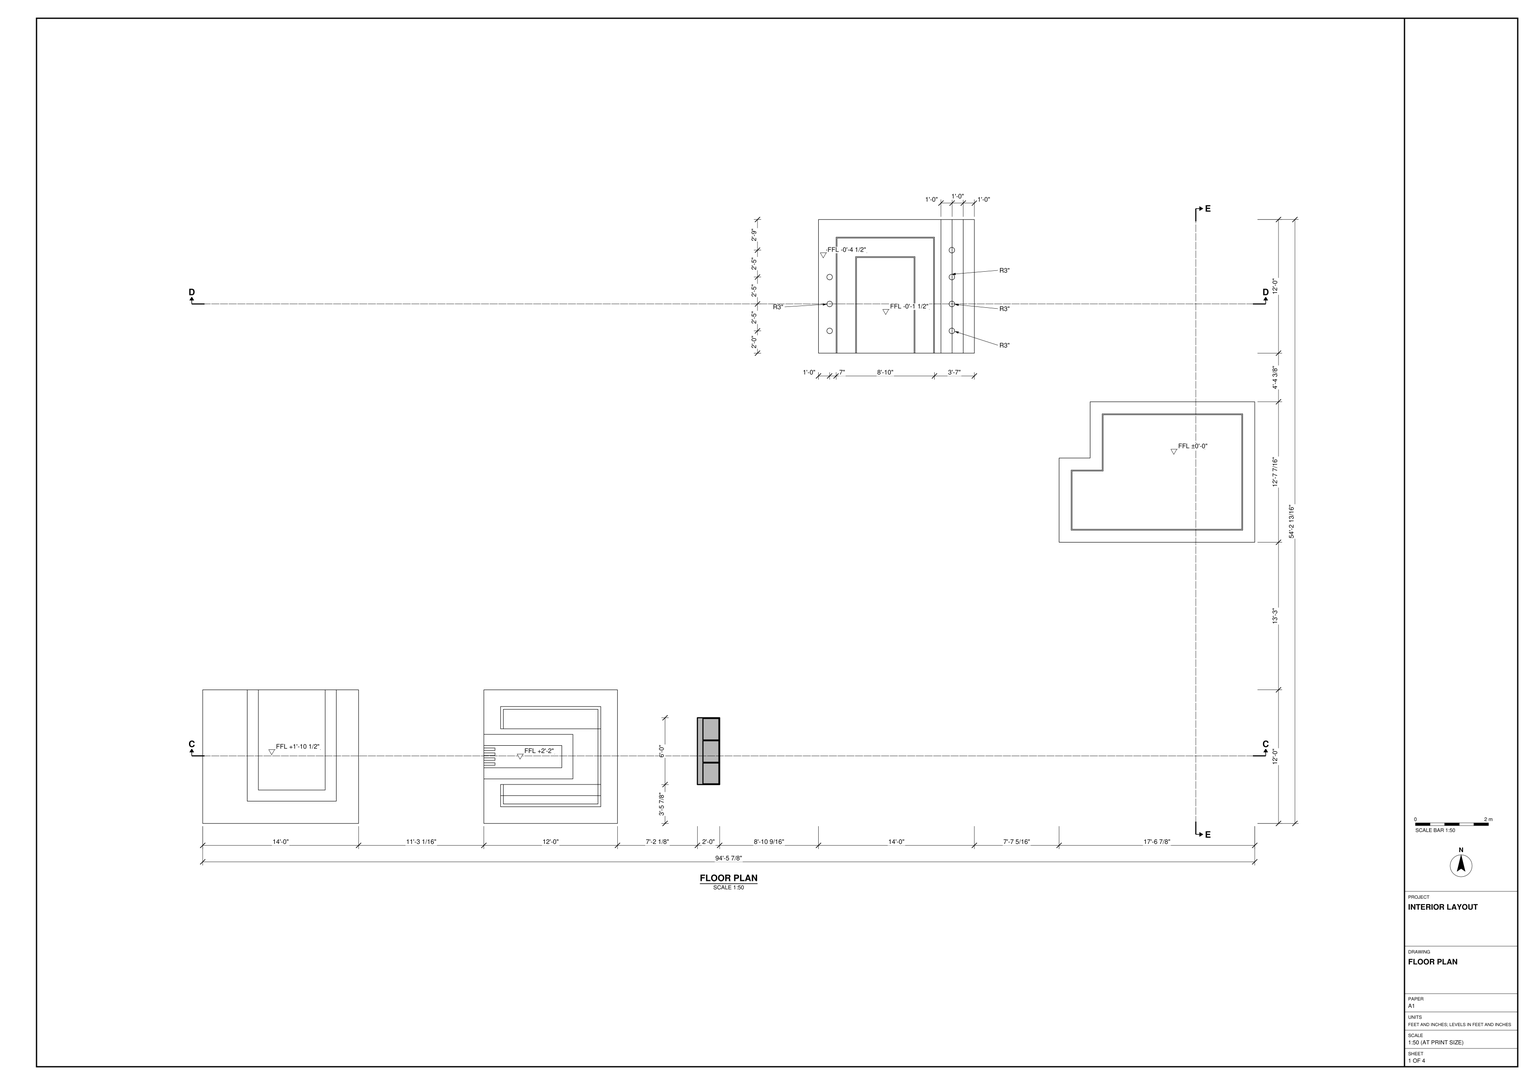
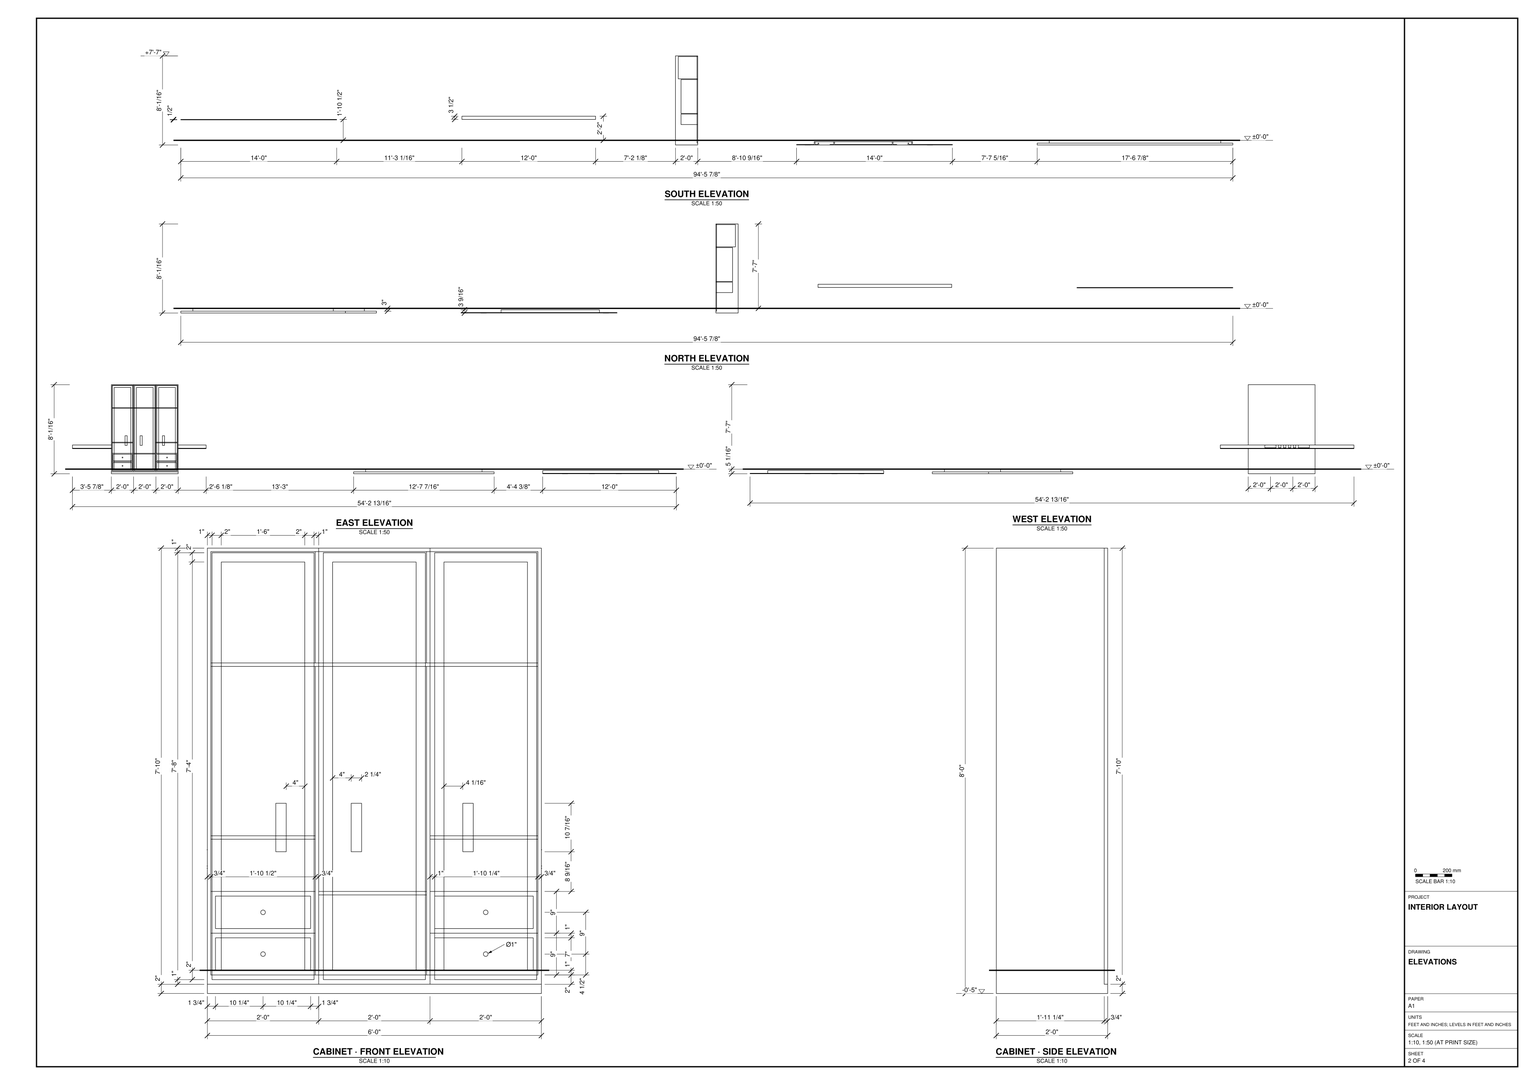
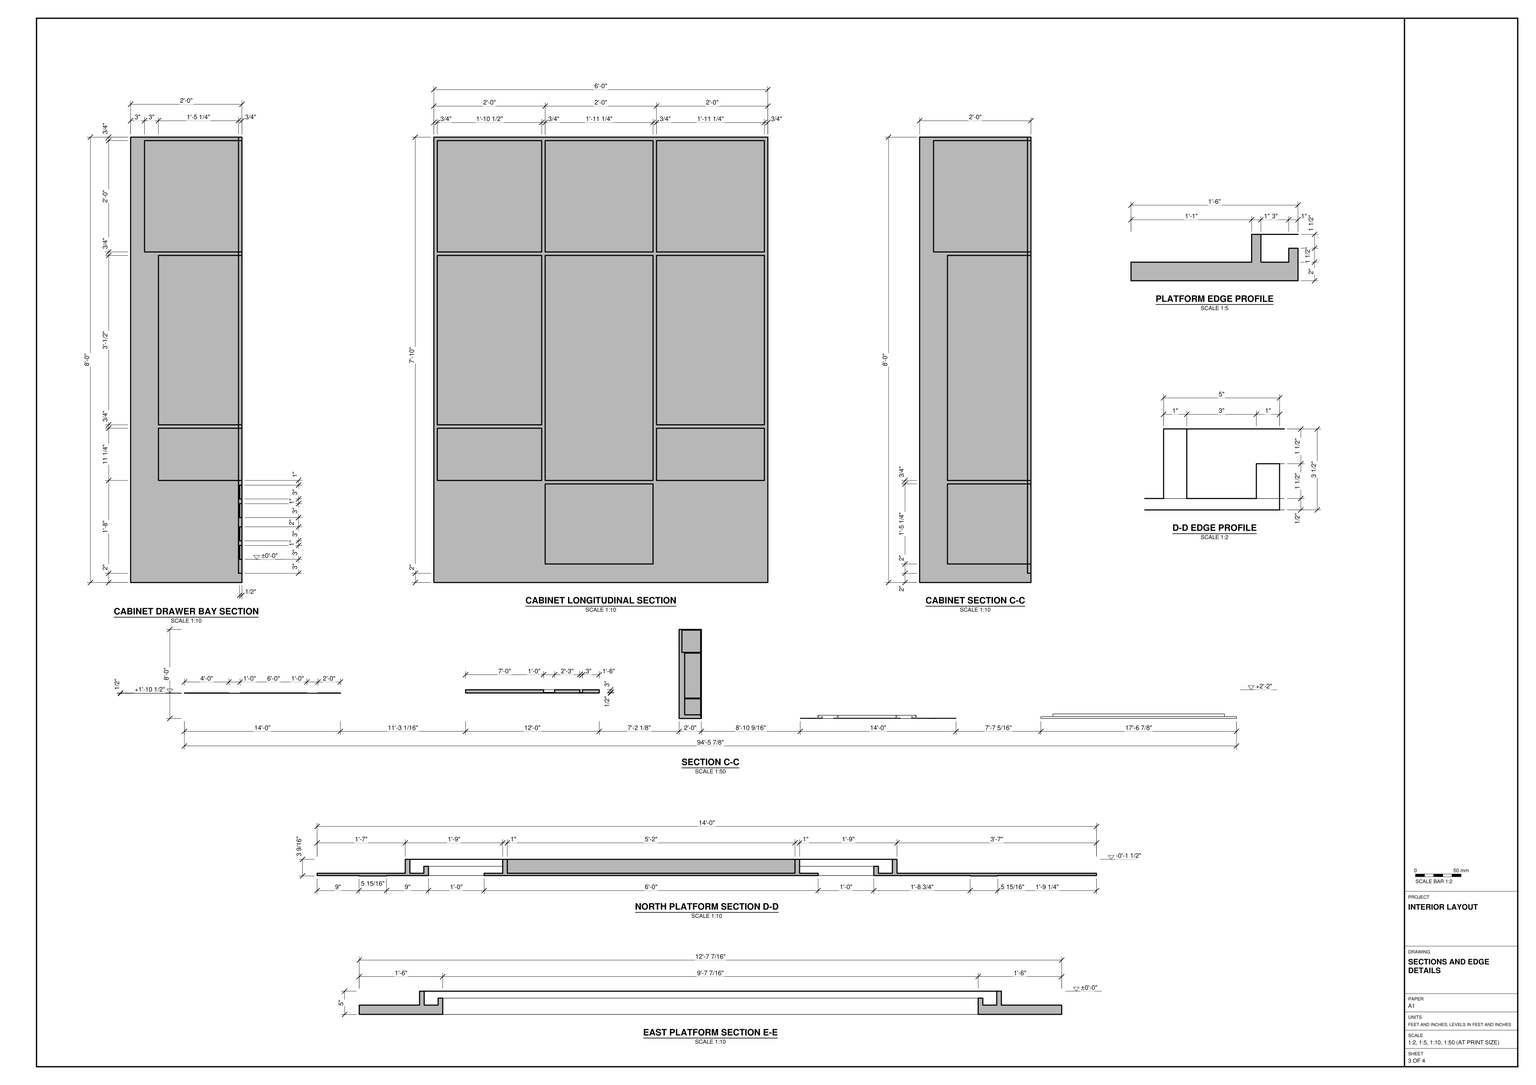
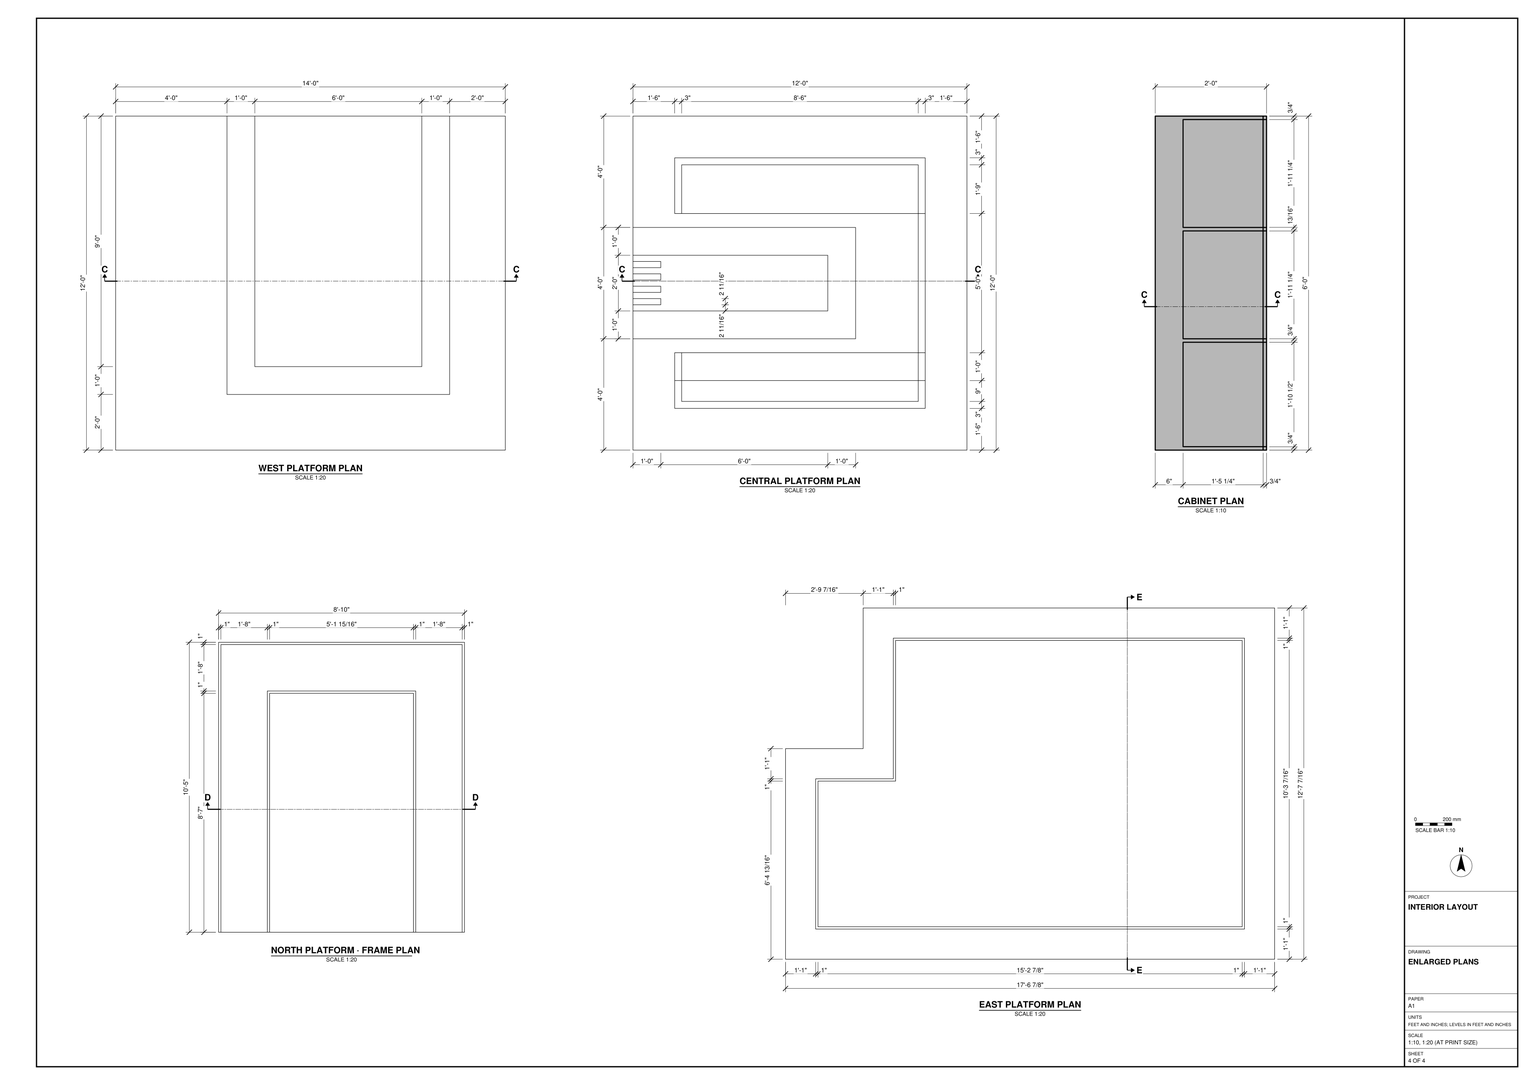
Build the interior layout in SketchUp from task_files/diagram_01.pdf. Work in feet and inches. Use ±0'-0" as the ground-floor datum. The complete layout measures 94'-5 7/8" east to west, 54'-2 13/16" north to south and 8'-1/16" from its lowest to its highest point.

Follow the floor plan for placement, keeping the gaps between pieces. Along the south row, model the rectangular platform with the U-shaped outline, the square platform with nested bands, and the tall cabinet with its front facing east. Set the platforms at their marked elevations rather than placing their undersides on the datum. Use the cabinet elevations for the framed fronts, pulls and lower drawers, and the sections for the carcass, shelf thicknesses and compartment divisions.

Farther north, reproduce the rectangular platform with its nested outlines, parallel strips and circular details. Give the east platform its stepped footprint and follow the step with the inset border. Use sections D-D and E-E and the enlarged edge details to model the changes in height across both platforms. Keep each platform and the cabinet as separate groups or components, and use components for repeated parts. Any decor or loose items shown may be represented by suitable library components. Save one SketchUp model as output_files/platform_layout_and_three_bay_storage_cabinet.skp.

# SketchUp Ruby script. Lengths in inches.
U = 1.inch
M = Sketchup.active_model
def pt(a) = Geom::Point3d.new(a.map { |v| v * U })
def face(e, loops, mat)
  f = e.add_face(loops[0].map { |a| pt(a) })
  loops[1..].each { |l| e.add_face(l.map { |a| pt(a) }).erase! }
  f.material = f.back_material = mat if mat
  f
end
# faces: each face lists its corners as indices into pts; further lists are holes
def faces(e, pts, list, mat = nil) = list.each { |f| face(e, (f[0].is_a?(Array) ? f : [f]).map { |l| l.map { |i| pts[i] } }, mat) }
# xy, xz, yz: faces in a plane at the given z, y or x. An outline is a flat list of corners, or four numbers for a rectangle; further outlines are holes
def ring(l) = l.size == 4 ? [[l[0], l[1]], [l[2], l[1]], [l[2], l[3]], [l[0], l[3]]] : l.each_slice(2).to_a
def flat(e, list, mat, &to3) = list.each { |f| face(e, (f[0].is_a?(Array) ? f : [f]).map { |l| ring(l).map { |u, v| to3.(u, v) } }, mat) }
def xy(e, z, list, mat = nil) = flat(e, list, mat) { |x, y| [x, y, z] }
def xz(e, y, list, mat = nil) = flat(e, list, mat) { |x, z| [x, y, z] }
def yz(e, x, list, mat = nil) = flat(e, list, mat) { |y, z| [x, y, z] }
def lines(e, pts, list) = list.each { |a, b| e.add_line(pt(pts[a]), pt(pts[b])) }
# prism: a flat outline (further loops are holes) pulled along v
def prism(e, loops, v, mat = nil)
  f = face(e, loops, mat); d = Geom::Vector3d.new(v.map { |x| x * U })
  f.pushpull(f.normal.samedirection?(d) ? d.length : -d.length)
end
def box(e, o, s, mat = nil) = prism(e, [[o, [o[0] + s[0], o[1], o[2]], [o[0] + s[0], o[1] + s[1], o[2]], [o[0], o[1] + s[1], o[2]]]], [0, 0, s[2]], mat)
def at(x, y, z, deg = 0) = Geom::Transformation.translation(pt([x, y, z])) * Geom::Transformation.rotation(ORIGIN, Z_AXIS, deg.degrees)
def axes(o, x, y, z) = Geom::Transformation.new([*x, 0, *y, 0, *z, 0, *pt(o).to_a, 1])
def part(name) = M.definitions.add(name)
# library, detail: a bought-in or finely detailed component or shape, given as its bounding box
def library(name, o, s) = part(name).tap { |d| box(d.entities, o, s) }
def detail(e, o, s) = box(e.add_group.entities, o, s)
def put(e, d, t, mat = nil) = e.add_instance(d, t).tap { |i| i.material = mat if mat }
def group(e, t, mat = nil) = e.add_group.tap { |g| g.transformation = t; g.material = mat if mat }.entities
root = M.entities
xy(root,-0.08,[[675.99,527.85,675.7,527.86,675.2,527.88,674.45,528.11,673.79,528.52,673.26,529.09,672.89,529.78,672.71,530.55,672.74,531.33,672.97,532.08,673.38,532.74,673.95,533.28,674.65,533.65,675.41,533.82,675.7,533.8125,676.19,533.8,676.94,533.57,677.6,533.15,678.14,532.58,678.51,531.89,678.68,531.125,678.66,530.34,678.43,529.59,678.01,528.93,677.44,528.4,676.75,528.03],[807.7,527.85,806.95,527.88,806.2,528.11,805.54,528.52,805.01,529.09,804.64,529.78,804.46,530.55,804.49,531.33,804.72,532.08,805.13,532.74,805.7,533.28,806.4,533.65,807.16,533.82,807.45,533.8125,807.7,533.8,807.94,533.8,808.69,533.57,809.35,533.15,809.89,532.58,810.26,531.89,810.43,531.125,810.41,530.34,810.18,529.59,809.76,528.93,809.19,528.4,808.5,528.03,807.74,527.85],[675.95,556.85,675.2,556.88,674.45,557.11,673.79,557.52,673.26,558.09,672.89,558.78,672.71,559.55,672.74,560.33,672.97,561.08,673.38,561.74,673.95,562.28,674.65,562.65,675.41,562.82,675.7,562.8125,675.95,562.8,676.19,562.8,676.94,562.57,677.6,562.15,678.14,561.58,678.51,560.89,678.68,560.125,678.66,559.34,678.43,558.59,678.01,557.93,677.44,557.4,676.75,557.03,675.99,556.85],[807.7,556.85,806.95,556.88,806.2,557.11,805.54,557.52,805.01,558.09,804.64,558.78,804.46,559.55,804.49,560.33,804.72,561.08,805.13,561.74,805.7,562.28,806.4,562.65,807.16,562.82,807.45,562.8125,807.7,562.8,807.94,562.8,808.69,562.57,809.35,562.15,809.89,561.58,810.26,560.89,810.43,560.125,810.41,559.34,810.18,558.59,809.76,557.93,809.19,557.4,808.5,557.03,807.74,556.85],[675.95,585.85,675.7,585.86,675.41,585.87,675.2,585.88,674.45,586.11,673.79,586.52,673.26,587.09,672.89,587.78,672.71,588.55,672.74,589.33,672.97,590.08,673.38,590.74,673.95,591.28,674.65,591.65,675.41,591.82,675.7,591.8125,675.95,591.8,676.19,591.8,676.94,591.57,677.6,591.15,678.14,590.58,678.51,589.89,678.68,589.125,678.66,588.34,678.43,587.59,678.01,586.93,677.44,586.4,676.75,586.03,675.99,585.85],
  [807.7,585.85,807.45,585.86,807.16,585.87,806.95,585.88,806.2,586.11,805.54,586.52,805.01,587.09,804.64,587.78,804.46,588.55,804.49,589.33,804.72,590.08,805.13,590.74,805.7,591.28,806.4,591.65,807.16,591.82,807.45,591.8125,807.7,591.8,807.94,591.8,808.69,591.57,809.35,591.15,809.89,590.58,810.26,589.89,810.43,589.125,810.41,588.34,810.18,587.59,809.76,586.93,809.19,586.4,808.5,586.03,807.74,585.85]])
xy(root,0,[[[663.7,506.84,663.7,650.84,795.7,650.84,795.7,506.84,783.7,506.84,783.7,626.84,687.7,626.84,687.7,506.84],[675.95,556.85,675.99,556.85,676.75,557.03,677.44,557.4,678.01,557.93,678.43,558.59,678.66,559.34,678.68,560.125,678.51,560.89,678.14,561.58,677.6,562.15,676.94,562.57,676.19,562.8,675.95,562.8,675.7,562.8125,675.41,562.82,674.65,562.65,673.95,562.28,673.38,561.74,672.97,561.08,672.74,560.33,672.71,559.55,672.89,558.78,673.26,558.09,673.79,557.52,674.45,557.11,675.2,556.88],[675.99,527.85,676.75,528.03,677.44,528.4,678.01,528.93,678.43,529.59,678.66,530.34,678.68,531.125,678.51,531.89,678.14,532.58,677.6,533.15,676.94,533.57,676.19,533.8,675.7,533.8125,675.41,533.82,674.65,533.65,673.95,533.28,673.38,532.74,672.97,532.08,672.74,531.33,672.71,530.55,672.89,529.78,673.26,529.09,673.79,528.52,674.45,528.11,675.2,527.88,675.7,527.86],[675.95,614.85,675.99,614.85,676.75,615.03,677.44,615.4,678.01,615.93,678.43,616.59,678.66,617.34,678.68,618.125,678.51,618.89,678.14,619.58,677.6,620.15,676.94,620.57,676.19,620.8,675.95,620.8,675.7,620.8125,675.41,620.82,674.65,620.65,673.95,620.28,673.38,619.74,672.97,619.08,672.74,618.33,672.71,617.55,672.89,616.78,673.26,616.09,673.79,615.52,674.45,615.11,675.2,614.88,675.41,614.87,675.7,614.86],[675.95,585.85,675.99,585.85,676.75,586.03,677.44,586.4,678.01,586.93,678.43,587.59,678.66,588.34,678.68,589.125,678.51,589.89,678.14,590.58,677.6,591.15,676.94,591.57,676.19,591.8,675.95,591.8,675.7,591.8125,675.41,591.82,674.65,591.65,673.95,591.28,673.38,590.74,672.97,590.08,672.74,589.33,672.71,588.55,672.89,587.78,673.26,587.09,673.79,586.52,674.45,586.11,675.2,585.88,675.41,585.87,675.7,585.86]],[699.7,506.84,771.7,614.84],[[795.7,506.84,819.7,650.84],[807.7,556.85,807.74,556.85,808.5,557.03,809.19,557.4,809.76,557.93,810.18,558.59,810.41,559.34,810.43,560.125,810.26,560.89,809.89,561.58,809.35,562.15,808.69,562.57,807.94,562.8,807.7,562.8,807.45,562.8125,807.16,562.82,806.4,562.65,805.7,562.28,805.13,561.74,804.72,561.08,804.49,560.33,804.46,559.55,804.64,558.78,805.01,558.09,805.54,557.52,806.2,557.11,806.95,556.88],[807.7,585.85,807.74,585.85,808.5,586.03,809.19,586.4,809.76,586.93,810.18,587.59,810.41,588.34,810.43,589.125,810.26,589.89,809.89,590.58,809.35,591.15,808.69,591.57,807.94,591.8,807.7,591.8,807.45,591.8125,807.16,591.82,806.4,591.65,805.7,591.28,805.13,590.74,804.72,590.08,804.49,589.33,804.46,588.55,804.64,587.78,805.01,587.09,805.54,586.52,806.2,586.11,806.95,585.88,807.16,585.87,807.45,585.86],[807.7,614.85,807.74,614.85,808.5,615.03,809.19,615.4,809.76,615.93,810.18,616.59,810.41,617.34,810.43,618.125,810.26,618.89,809.89,619.58,809.35,620.15,808.69,620.57,807.94,620.8,807.7,620.8,807.45,620.8125,807.16,620.82,806.4,620.65,805.7,620.28,805.13,619.74,804.72,619.08,804.49,618.33,804.46,617.55,804.64,616.78,805.01,616.09,805.54,615.52,806.2,615.11,806.95,614.88,807.16,614.87,807.45,614.86],[807.7,527.85,807.74,527.85,808.5,528.03,809.19,528.4,809.76,528.93,810.18,529.59,810.41,530.34,810.43,531.125,810.26,531.89,809.89,532.58,809.35,533.15,808.69,533.57,807.94,533.8,807.7,533.8,807.45,533.8125,807.16,533.82,806.4,533.65,805.7,533.28,805.13,532.74,804.72,532.08,804.49,531.33,804.46,530.55,804.64,529.78,805.01,529.09,805.54,528.52,806.2,528.11,806.95,527.88]],[819.7,506.84,831.7,650.84]])
xy(root,0.04,[[807.7,614.85,807.45,614.86,807.16,614.87,806.95,614.88,806.2,615.11,805.54,615.52,805.01,616.09,804.64,616.78,804.46,617.55,804.49,618.33,804.72,619.08,805.13,619.74,805.7,620.28,806.4,620.65,807.16,620.82,807.45,620.8125,807.7,620.8,807.94,620.8,808.69,620.57,809.35,620.15,809.89,619.58,810.26,618.89,810.43,618.125,810.41,617.34,810.18,616.59,809.76,615.93,809.19,615.4,808.5,615.03,807.74,614.85]])
xy(root,0.49,[[663.7,506.84,682.7,506.84,682.7,631.84,788.7,631.84,788.7,506.84,807.7,506.84,807.7,650.84,663.7,650.84],[683.7,506.84,686.7,506.84,686.7,627.84,784.7,627.84,784.7,506.84,787.7,506.84,787.7,630.84,683.7,630.84],[699.7,506.84,700.7,506.84,700.7,613.84,770.7,613.84,770.7,506.84,771.7,506.84,771.7,614.84,699.7,614.84],[700.7,506.84,703.7,506.84,703.7,610.84,767.7,610.84,767.7,506.84,770.7,506.84,770.7,613.84,700.7,613.84],[704.7,506.84,766.7,609.84],
  [807.7,506.84,831.7,650.84]])
xy(root,1.99,[[686.7,506.84,687.7,506.84,687.7,626.84,783.7,626.84,783.7,506.84,784.7,506.84,784.7,627.84,686.7,627.84]])
xy(root,3.49,[[682.7,506.84,683.7,506.84,683.7,630.84,787.7,630.84,787.7,506.84,788.7,506.84,788.7,631.84,682.7,631.84],[683.7,506.84,703.7,506.84,703.7,610.84,767.7,610.84,767.7,506.84,787.7,506.84,787.7,630.84,683.7,630.84],[703.7,506.84,704.7,506.84,704.7,609.84,766.7,609.84,766.7,506.84,767.7,506.84,767.7,610.84,703.7,610.84],[704.7,506.84,766.7,609.84]])
xy(root,27.49,[[0,0,168,0,168,144,144,144,144,24,48,24,48,144,0,144],[303.04,0,447.04,144],[60,36,132,144]])
xy(root,27.98,[[321.04,18,429.04,18,429.04,30,426.04,30,426.04,21,324.04,21,324.04,30,321.04,30],[324.04,21,426.04,30],[321.04,30,324.04,42],[324.04,30,426.04,42],[426.04,30,429.04,42],
  [426.04,42,429.04,102],[303.04,48,399.04,48,399.04,96,303.04,96,303.04,84,387.04,84,387.04,60,303.04,60],[303.04,62.67,315.04,65.33],[303.04,68,315.04,70.67],[303.04,73.33,315.04,76],
  [303.04,78.67,315.04,81.33],[321.04,102,324.04,102,324.04,123,426.04,123,426.04,102,429.04,102,429.04,126,321.04,126],[324.04,102,426.04,123]])
xy(root,30.98,[[[303.04,0,447.04,0,447.04,144,303.04,144,303.04,96,399.04,96,399.04,48,303.04,48],[321.04,18,321.04,42,426.04,42,426.04,102,321.04,102,321.04,126,429.04,126,429.04,18]],[303.04,60,387.04,60,387.04,84,303.04,84,303.04,81.33,315.04,81.33,315.04,78.67,303.04,78.67,303.04,76,315.04,76,315.04,73.33,303.04,73.33,303.04,70.67,315.04,70.67,315.04,68,303.04,68,303.04,65.33,315.04,65.33,315.04,62.67,303.04,62.67]])
xz(root,0,[[0,27,168,27.49],[303.04,27.49,447.04,30.98]])
xz(root,18,[[321.04,27.98,429.04,30.98]])
xz(root,42,[[321.04,27.98,324.04,30.98],[324.04,27.98,426.04,30.98]])
xz(root,48,[[303.04,27.98,399.04,30.98]])
xz(root,60,[[303.04,27.98,387.04,30.98]])
xz(root,62.67,[[303.04,27.98,315.04,30.98]])
xz(root,65.33,[[303.04,27.98,315.04,30.98]])
xz(root,68,[[303.04,27.98,315.04,30.98]])
xz(root,70.67,[[303.04,27.98,315.04,30.98]])
xz(root,73.33,[[303.04,27.98,315.04,30.98]])
xz(root,76,[[303.04,27.98,315.04,30.98]])
xz(root,78.67,[[303.04,27.98,315.04,30.98]])
xz(root,81.33,[[303.04,27.98,315.04,30.98]])
xz(root,84,[[303.04,27.98,387.04,30.98]])
xz(root,96,[[303.04,27.98,399.04,30.98]])
xz(root,102,[[321.04,27.98,324.04,30.98],[324.04,27.98,426.04,30.98]])
xz(root,126,[[321.04,27.98,429.04,30.98]])
xz(root,144,[[0,27,168,27.49],[303.04,27.49,447.04,30.98]])
xz(root,506.84,[[663.7,0,687.7,0,687.7,1.99,686.7,1.99,686.7,0.49,683.7,0.49,683.7,3.49,682.7,3.49,682.7,0.49,663.7,0.49],[687.7,0,699.7,0,699.7,0.49,703.7,0.49,703.7,3.49,683.7,3.49,683.7,0.49,686.7,0.49,686.7,1.99,687.7,1.99],[699.7,0,771.7,0,771.7,0.49,767.7,0.49,767.7,3.49,766.7,3.49,766.7,0.49,704.7,0.49,704.7,3.49,703.7,3.49,703.7,0.49,699.7,0.49],[771.7,0,783.7,0,783.7,1.99,784.7,1.99,784.7,0.49,787.7,0.49,787.7,3.49,767.7,3.49,767.7,0.49,771.7,0.49],[783.7,0,807.7,0,807.7,0.49,788.7,0.49,788.7,3.49,787.7,3.49,787.7,0.49,784.7,0.49,784.7,1.99,783.7,1.99],
  [807.7,0,831.7,0.49],[704.7,0.49,766.7,3.49]])
xz(root,527.85,[[807.7,-0.08,807.74,0]])
xz(root,533.8,[[807.7,-0.08,807.94,0]])
xz(root,556.85,[[675.95,-0.08,675.99,0],[807.7,-0.08,807.74,0]])
xz(root,562.8,[[675.95,-0.08,676.19,0],[807.7,-0.08,807.94,0]])
xz(root,585.85,[[675.95,-0.08,675.99,0],[807.7,-0.08,807.74,0]])
xz(root,591.8,[[675.95,-0.08,676.19,0],[807.7,-0.08,807.94,0]])
xz(root,609.84,[[704.7,0.49,766.7,3.49]])
xz(root,610.84,[[703.7,0.49,767.7,3.49]])
xz(root,614.84,[[699.7,0,771.7,0.49]])
xz(root,614.85,[[675.95,0,675.99,0.04],[807.7,0,807.74,0.04]])
xz(root,620.8,[[675.95,0,676.19,0.04],[807.7,0,807.94,0.04]])
xz(root,626.84,[[687.7,0,783.7,1.99]])
xz(root,627.84,[[686.7,0.49,784.7,1.99]])
xz(root,630.84,[[683.7,0.49,787.7,3.49]])
xz(root,631.84,[[682.7,0.49,788.7,3.49]])
xz(root,650.84,[[663.7,0,807.7,0.49],[807.7,0,831.7,0.49]])
yz(root,0,[[0,27,144,27.49]])
yz(root,168,[[0,27,144,27.49]])
yz(root,303.04,[[0,27.49,0,30.98,48,30.98,48,27.98,60,27.98,60,30.98,62.67,30.98,62.67,27.98,65.33,27.98,65.33,30.98,68,30.98,68,27.98,70.67,27.98,70.67,30.98,73.33,30.98,73.33,27.98,76,27.98,76,30.98,78.67,30.98,78.67,27.98,81.33,27.98,81.33,30.98,84,30.98,84,27.98,96,27.98,96,30.98,144,30.98,144,27.49]])
yz(root,315.04,[[62.67,27.98,65.33,30.98],[68,27.98,70.67,30.98],[73.33,27.98,76,30.98],[78.67,27.98,81.33,30.98]])
yz(root,321.04,[[18,27.98,42,30.98],[102,27.98,126,30.98]])
yz(root,387.04,[[60,27.98,84,30.98]])
yz(root,399.04,[[48,27.98,96,30.98]])
yz(root,426.04,[[42,27.98,102,30.98]])
yz(root,429.04,[[18,27.98,42,30.98],[42,27.98,102,30.98],[102,27.98,126,30.98]])
yz(root,447.04,[[0,27.49,144,30.98]])
yz(root,663.7,[[506.84,0,650.84,0.49]])
yz(root,682.7,[[506.84,0.49,631.84,3.49]])
yz(root,683.7,[[506.84,0.49,630.84,3.49]])
yz(root,686.7,[[506.84,0.49,627.84,1.99]])
yz(root,687.7,[[506.84,0,626.84,1.99]])
yz(root,699.7,[[506.84,0,614.84,0.49]])
yz(root,703.7,[[506.84,0.49,610.84,3.49]])
yz(root,704.7,[[506.84,0.49,609.84,3.49]])
yz(root,766.7,[[506.84,0.49,609.84,3.49]])
yz(root,767.7,[[506.84,0.49,610.84,3.49]])
yz(root,771.7,[[506.84,0,614.84,0.49]])
yz(root,783.7,[[506.84,0,626.84,1.99]])
yz(root,784.7,[[506.84,0.49,627.84,1.99]])
yz(root,787.7,[[506.84,0.49,630.84,3.49]])
yz(root,788.7,[[506.84,0.49,631.84,3.49]])
yz(root,831.7,[[506.84,0,650.84,0.49]])
p = [[675.2,527.88,0],[674.45,528.11,0],[674.45,528.11,-0.08],[675.2,527.88,-0.08],[675.7,527.86,0],[675.7,527.86,-0.08],
  [675.99,527.85,0],[675.99,527.85,-0.08],[676.75,528.03,0],[676.75,528.03,-0.08],[806.95,527.88,0],[806.2,528.11,0],
  [806.2,528.11,-0.08],[806.95,527.88,-0.08],[807.45,527.86,0],[807.45,527.86,-0.08],[807.7,527.85,0],[807.7,527.85,-0.08],
  [808.5,528.03,0],[807.74,527.85,0],[807.74,527.85,-0.08],[808.5,528.03,-0.08],[677.44,528.4,0],[677.44,528.4,-0.08],
  [809.19,528.4,0],[809.19,528.4,-0.08],[673.79,528.52,0],[673.79,528.52,-0.08],[805.54,528.52,0],[805.54,528.52,-0.08],
  [678.01,528.93,0],[678.01,528.93,-0.08],[809.76,528.93,0],[809.76,528.93,-0.08],[673.26,529.09,0],[673.26,529.09,-0.08],
  [805.01,529.09,0],[805.01,529.09,-0.08],[678.43,529.59,0],[678.43,529.59,-0.08],[810.18,529.59,0],[810.18,529.59,-0.08],
  [672.89,529.78,0],[672.89,529.78,-0.08],[804.64,529.78,0],[804.64,529.78,-0.08],[678.66,530.34,0],[678.66,530.34,-0.08],
  [810.41,530.34,0],[810.41,530.34,-0.08],[672.71,530.55,0],[672.71,530.55,-0.08],[804.46,530.55,0],[804.46,530.55,-0.08],
  [678.68,531.125,0],[678.68,531.125,-0.08],[810.43,531.125,0],[810.43,531.125,-0.08],[672.74,531.33,0],[672.74,531.33,-0.08],
  [804.49,531.33,0],[804.49,531.33,-0.08],[678.51,531.89,0],[678.51,531.89,-0.08],[810.26,531.89,0],[810.26,531.89,-0.08],
  [672.97,532.08,0],[672.97,532.08,-0.08],[804.72,532.08,0],[804.72,532.08,-0.08],[678.14,532.58,0],[678.14,532.58,-0.08],
  [809.89,532.58,0],[809.89,532.58,-0.08],[673.38,532.74,0],[673.38,532.74,-0.08],[805.13,532.74,0],[805.13,532.74,-0.08],
  [677.6,533.15,0],[677.6,533.15,-0.08],[809.35,533.15,0],[809.35,533.15,-0.08],[673.95,533.28,0],[673.95,533.28,-0.08],
  [805.7,533.28,0],[805.7,533.28,-0.08],[676.94,533.57,0],[676.94,533.57,-0.08],[808.69,533.57,0],[808.69,533.57,-0.08],
  [674.65,533.65,0],[674.65,533.65,-0.08],[806.4,533.65,0],[806.4,533.65,-0.08],[675.41,533.82,0],[675.41,533.82,-0.08],
  [676.19,533.8,0],[676.19,533.8,-0.08],[807.16,533.82,0],[807.16,533.82,-0.08],[807.94,533.8,0],[807.94,533.8,-0.08],
  [675.7,533.8125,0],[675.7,533.8125,-0.08],[807.45,533.8125,0],[807.45,533.8125,-0.08],[807.7,533.8,0],[807.7,533.8,-0.08],
  [675.2,556.88,0],[674.45,557.11,0],[674.45,557.11,-0.08],[675.2,556.88,-0.08],[675.7,556.86,0],[675.7,556.86,-0.08],
  [675.95,556.85,0],[675.95,556.85,-0.08],[676.75,557.03,0],[675.99,556.85,0],[675.99,556.85,-0.08],[676.75,557.03,-0.08],
  [806.95,556.88,0],[806.2,557.11,0],[806.2,557.11,-0.08],[806.95,556.88,-0.08],[807.45,556.86,0],[807.45,556.86,-0.08],
  [807.7,556.85,0],[807.7,556.85,-0.08],[808.5,557.03,0],[807.74,556.85,0],[807.74,556.85,-0.08],[808.5,557.03,-0.08],
  [677.44,557.4,0],[677.44,557.4,-0.08],[809.19,557.4,0],[809.19,557.4,-0.08],[673.79,557.52,0],[673.79,557.52,-0.08],
  [805.54,557.52,0],[805.54,557.52,-0.08],[678.01,557.93,0],[678.01,557.93,-0.08],[809.76,557.93,0],[809.76,557.93,-0.08],
  [673.26,558.09,0],[673.26,558.09,-0.08],[805.01,558.09,0],[805.01,558.09,-0.08],[678.43,558.59,0],[678.43,558.59,-0.08],
  [810.18,558.59,0],[810.18,558.59,-0.08],[672.89,558.78,0],[672.89,558.78,-0.08],[804.64,558.78,0],[804.64,558.78,-0.08],
  [678.66,559.34,0],[678.66,559.34,-0.08],[810.41,559.34,0],[810.41,559.34,-0.08],[672.71,559.55,0],[672.71,559.55,-0.08],
  [804.46,559.55,0],[804.46,559.55,-0.08],[678.68,560.125,0],[678.68,560.125,-0.08],[810.43,560.125,0],[810.43,560.125,-0.08],
  [672.74,560.33,0],[672.74,560.33,-0.08],[804.49,560.33,0],[804.49,560.33,-0.08],[678.51,560.89,0],[678.51,560.89,-0.08],
  [810.26,560.89,0],[810.26,560.89,-0.08],[672.97,561.08,0],[672.97,561.08,-0.08],[804.72,561.08,0],[804.72,561.08,-0.08],
  [678.14,561.58,0],[678.14,561.58,-0.08],[809.89,561.58,0],[809.89,561.58,-0.08],[673.38,561.74,0],[673.38,561.74,-0.08],
  [805.13,561.74,0],[805.13,561.74,-0.08],[677.6,562.15,0],[677.6,562.15,-0.08],[809.35,562.15,0],[809.35,562.15,-0.08],
  [673.95,562.28,0],[673.95,562.28,-0.08],[805.7,562.28,0],[805.7,562.28,-0.08],[676.94,562.57,0],[676.94,562.57,-0.08],
  [808.69,562.57,0],[808.69,562.57,-0.08],[674.65,562.65,0],[674.65,562.65,-0.08],[806.4,562.65,0],[806.4,562.65,-0.08],
  [675.41,562.82,0],[675.41,562.82,-0.08],[676.19,562.8,0],[676.19,562.8,-0.08],[807.16,562.82,0],[807.16,562.82,-0.08],
  [807.94,562.8,0],[807.94,562.8,-0.08],[675.7,562.8125,0],[675.7,562.8125,-0.08],[675.95,562.8,0],[675.95,562.8,-0.08],
  [807.45,562.8125,0],[807.45,562.8125,-0.08],[807.7,562.8,0],[807.7,562.8,-0.08],[675.2,585.88,0],[674.45,586.11,0],
  [674.45,586.11,-0.08],[675.2,585.88,-0.08],[675.41,585.87,0],[675.41,585.87,-0.08],[675.7,585.86,0],[675.7,585.86,-0.08],
  [675.95,585.85,0],[675.95,585.85,-0.08],[676.75,586.03,0],[675.99,585.85,0],[675.99,585.85,-0.08],[676.75,586.03,-0.08],
  [806.95,585.88,0],[806.2,586.11,0],[806.2,586.11,-0.08],[806.95,585.88,-0.08],[807.16,585.87,0],[807.16,585.87,-0.08],
  [807.45,585.86,0],[807.45,585.86,-0.08],[807.7,585.85,0],[807.7,585.85,-0.08],[808.5,586.03,0],[807.74,585.85,0],
  [807.74,585.85,-0.08],[808.5,586.03,-0.08],[677.44,586.4,0],[677.44,586.4,-0.08],[809.19,586.4,0],[809.19,586.4,-0.08],
  [673.79,586.52,0],[673.79,586.52,-0.08],[805.54,586.52,0],[805.54,586.52,-0.08],[678.01,586.93,0],[678.01,586.93,-0.08],
  [809.76,586.93,0],[809.76,586.93,-0.08],[673.26,587.09,0],[673.26,587.09,-0.08],[805.01,587.09,0],[805.01,587.09,-0.08],
  [678.43,587.59,0],[678.43,587.59,-0.08],[810.18,587.59,0],[810.18,587.59,-0.08],[672.89,587.78,0],[672.89,587.78,-0.08],
  [804.64,587.78,0],[804.64,587.78,-0.08],[678.66,588.34,0],[678.66,588.34,-0.08],[810.41,588.34,0],[810.41,588.34,-0.08],
  [672.71,588.55,0],[672.71,588.55,-0.08],[804.46,588.55,0],[804.46,588.55,-0.08],[678.68,589.125,0],[678.68,589.125,-0.08],
  [810.43,589.125,0],[810.43,589.125,-0.08],[672.74,589.33,0],[672.74,589.33,-0.08],[804.49,589.33,0],[804.49,589.33,-0.08],
  [678.51,589.89,0],[678.51,589.89,-0.08],[810.26,589.89,0],[810.26,589.89,-0.08],[672.97,590.08,0],[672.97,590.08,-0.08],
  [804.72,590.08,0],[804.72,590.08,-0.08],[678.14,590.58,0],[678.14,590.58,-0.08],[809.89,590.58,0],[809.89,590.58,-0.08],
  [673.38,590.74,0],[673.38,590.74,-0.08],[805.13,590.74,0],[805.13,590.74,-0.08],[677.6,591.15,0],[677.6,591.15,-0.08],
  [809.35,591.15,0],[809.35,591.15,-0.08],[673.95,591.28,0],[673.95,591.28,-0.08],[805.7,591.28,0],[805.7,591.28,-0.08],
  [676.94,591.57,0],[676.94,591.57,-0.08],[808.69,591.57,0],[808.69,591.57,-0.08],[674.65,591.65,0],[674.65,591.65,-0.08],
  [806.4,591.65,0],[806.4,591.65,-0.08],[675.41,591.82,0],[675.41,591.82,-0.08],[676.19,591.8,0],[676.19,591.8,-0.08],
  [807.16,591.82,0],[807.16,591.82,-0.08],[807.94,591.8,0],[807.94,591.8,-0.08],[675.7,591.8125,0],[675.7,591.8125,-0.08],
  [675.95,591.8,0],[675.95,591.8,-0.08],[807.45,591.8125,0],[807.45,591.8125,-0.08],[807.7,591.8,0],[807.7,591.8,-0.08],
  [675.2,614.88,0],[674.45,615.11,0],[674.45,615.11,0.04],[675.2,614.88,0.04],[675.41,614.87,0],[675.41,614.87,0.04],
  [675.7,614.86,0],[675.7,614.86,0.04],[675.95,614.85,0],[675.95,614.85,0.04],[676.75,615.03,0],[675.99,614.85,0],
  [675.99,614.85,0.04],[676.75,615.03,0.04],[806.95,614.88,0],[806.2,615.11,0],[806.2,615.11,0.04],[806.95,614.88,0.04],
  [807.16,614.87,0],[807.16,614.87,0.04],[807.45,614.86,0],[807.45,614.86,0.04],[807.7,614.85,0],[807.7,614.85,0.04],
  [808.5,615.03,0],[807.74,614.85,0],[807.74,614.85,0.04],[808.5,615.03,0.04],[677.44,615.4,0],[677.44,615.4,0.04],
  [809.19,615.4,0],[809.19,615.4,0.04],[673.79,615.52,0],[673.79,615.52,0.04],[805.54,615.52,0],[805.54,615.52,0.04],
  [678.01,615.93,0],[678.01,615.93,0.04],[809.76,615.93,0],[809.76,615.93,0.04],[673.26,616.09,0],[673.26,616.09,0.04],
  [805.01,616.09,0],[805.01,616.09,0.04],[678.43,616.59,0],[678.43,616.59,0.04],[810.18,616.59,0],[810.18,616.59,0.04],
  [672.89,616.78,0],[672.89,616.78,0.04],[804.64,616.78,0],[804.64,616.78,0.04],[678.66,617.34,0],[678.66,617.34,0.04],
  [810.41,617.34,0],[810.41,617.34,0.04],[672.71,617.55,0],[672.71,617.55,0.04],[804.46,617.55,0],[804.46,617.55,0.04],
  [678.68,618.125,0],[678.68,618.125,0.04],[810.43,618.125,0],[810.43,618.125,0.04],[672.74,618.33,0],[672.74,618.33,0.04],
  [804.49,618.33,0],[804.49,618.33,0.04],[678.51,618.89,0],[678.51,618.89,0.04],[810.26,618.89,0],[810.26,618.89,0.04],
  [672.97,619.08,0],[672.97,619.08,0.04],[804.72,619.08,0],[804.72,619.08,0.04],[678.14,619.58,0],[678.14,619.58,0.04],
  [809.89,619.58,0],[809.89,619.58,0.04],[673.38,619.74,0],[673.38,619.74,0.04],[805.13,619.74,0],[805.13,619.74,0.04],
  [677.6,620.15,0],[677.6,620.15,0.04],[809.35,620.15,0],[809.35,620.15,0.04],[673.95,620.28,0],[673.95,620.28,0.04],
  [805.7,620.28,0],[805.7,620.28,0.04],[676.94,620.57,0],[676.94,620.57,0.04],[808.69,620.57,0],[808.69,620.57,0.04],
  [674.65,620.65,0],[674.65,620.65,0.04],[806.4,620.65,0],[806.4,620.65,0.04],[675.41,620.82,0],[675.41,620.82,0.04],
  [676.19,620.8,0],[676.19,620.8,0.04],[807.16,620.82,0],[807.16,620.82,0.04],[807.94,620.8,0],[807.94,620.8,0.04],
  [675.7,620.8125,0],[675.7,620.8125,0.04],[675.95,620.8,0],[675.95,620.8,0.04],[807.45,620.8125,0],[807.45,620.8125,0.04],
  [807.7,620.8,0],[807.7,620.8,0.04]]
faces(root,p,[[0,1,2,3],[4,0,3,5],[6,4,5,7],[8,6,7,9],[10,11,12,13],[14,10,13,15],[16,14,15,17],[18,19,20,21],
  [22,8,9,23],[24,18,21,25],[1,26,27,2],[11,28,29,12],[30,22,23,31],[32,24,25,33],[26,34,35,27],[28,36,37,29],
  [38,30,31,39],[40,32,33,41],[34,42,43,35],[36,44,45,37],[46,38,39,47],[48,40,41,49],[42,50,51,43],[44,52,53,45],
  [54,46,47,55],[56,48,49,57],[50,58,59,51],[52,60,61,53],[62,54,55,63],[64,56,57,65],[58,66,67,59],[60,68,69,61],
  [70,62,63,71],[72,64,65,73],[66,74,75,67],[68,76,77,69],[78,70,71,79],[80,72,73,81],[74,82,83,75],[76,84,85,77],
  [86,78,79,87],[88,80,81,89],[82,90,91,83],[84,92,93,85],[90,94,95,91],[96,86,87,97],[92,98,99,93],[100,88,89,101],
  [94,102,103,95],[102,96,97,103],[98,104,105,99],[104,106,107,105],[108,109,110,111],[112,108,111,113],[114,112,113,115],[116,117,118,119],
  [120,121,122,123],[124,120,123,125],[126,124,125,127],[128,129,130,131],[132,116,119,133],[134,128,131,135],[109,136,137,110],[121,138,139,122],
  [140,132,133,141],[142,134,135,143],[136,144,145,137],[138,146,147,139],[148,140,141,149],[150,142,143,151],[144,152,153,145],[146,154,155,147],
  [156,148,149,157],[158,150,151,159],[152,160,161,153],[154,162,163,155],[164,156,157,165],[166,158,159,167],[160,168,169,161],[162,170,171,163],
  [172,164,165,173],[174,166,167,175],[168,176,177,169],[170,178,179,171],[180,172,173,181],[182,174,175,183],[176,184,185,177],[178,186,187,179],
  [188,180,181,189],[190,182,183,191],[184,192,193,185],[186,194,195,187],[196,188,189,197],[198,190,191,199],[192,200,201,193],[194,202,203,195],
  [200,204,205,201],[206,196,197,207],[202,208,209,203],[210,198,199,211],[204,212,213,205],[212,214,215,213],[208,216,217,209],[216,218,219,217],
  [220,221,222,223],[224,220,223,225],[226,224,225,227],[228,226,227,229],[230,231,232,233],[234,235,236,237],[238,234,237,239],[240,238,239,241],
  [242,240,241,243],[244,245,246,247],[248,230,233,249],[250,244,247,251],[221,252,253,222],[235,254,255,236],[256,248,249,257],[258,250,251,259],
  [252,260,261,253],[254,262,263,255],[264,256,257,265],[266,258,259,267],[260,268,269,261],[262,270,271,263],[272,264,265,273],[274,266,267,275],
  [268,276,277,269],[270,278,279,271],[280,272,273,281],[282,274,275,283],[276,284,285,277],[278,286,287,279],[288,280,281,289],[290,282,283,291],
  [284,292,293,285],[286,294,295,287],[296,288,289,297],[298,290,291,299],[292,300,301,293],[294,302,303,295],[304,296,297,305],[306,298,299,307],
  [300,308,309,301],[302,310,311,303],[312,304,305,313],[314,306,307,315],[308,316,317,309],[310,318,319,311],[316,320,321,317],[322,312,313,323],
  [318,324,325,319],[326,314,315,327],[320,328,329,321],[328,330,331,329],[324,332,333,325],[332,334,335,333],[336,337,338,339],[340,336,339,341],
  [342,340,341,343],[344,342,343,345],[346,347,348,349],[350,351,352,353],[354,350,353,355],[356,354,355,357],[358,356,357,359],[360,361,362,363],
  [364,346,349,365],[366,360,363,367],[337,368,369,338],[351,370,371,352],[372,364,365,373],[374,366,367,375],[368,376,377,369],[370,378,379,371],
  [380,372,373,381],[382,374,375,383],[376,384,385,377],[378,386,387,379],[388,380,381,389],[390,382,383,391],[384,392,393,385],[386,394,395,387],
  [396,388,389,397],[398,390,391,399],[392,400,401,393],[394,402,403,395],[404,396,397,405],[406,398,399,407],[400,408,409,401],[402,410,411,403],
  [412,404,405,413],[414,406,407,415],[408,416,417,409],[410,418,419,411],[420,412,413,421],[422,414,415,423],[416,424,425,417],[418,426,427,419],
  [428,420,421,429],[430,422,423,431],[424,432,433,425],[426,434,435,427],[432,436,437,433],[438,428,429,439],[434,440,441,435],[442,430,431,443],
  [436,444,445,437],[444,446,447,445],[440,448,449,441],[448,450,451,449]])
detail(root,[533.16,41.91,0],[24,72,96])
g1 = group(root,at(556.41,89.91,2))
xy(g1,0,[[0,0,0.75,24]])
xy(g1,94,[[0,0,0.75,24]])
xz(g1,0,[[0,0,0.75,94]])
xz(g1,24,[[0,0,0.75,94]])
yz(g1,0,[[0,0,24,94]])
yz(g1,0.75,[[[0,0,24,94],[1,1,23,93]],[[1,1,23,93],[3,3,21,91]],[[3,3,21,91],[7.0625,28.5625,9.3125,39]],[7.0625,28.5625,9.3125,39]])
g2 = group(root,at(556.41,65.91,2))
xy(g2,0,[[0,0,0.75,24]])
xy(g2,94,[[0,0,0.75,24]])
xz(g2,0,[[0,0,0.75,94]])
xz(g2,24,[[0,0,0.75,94]])
yz(g2,0,[[0,0,24,94]])
yz(g2,0.75,[[[0,0,24,94],[1,1,23,93]],[[1,1,23,93],[3,3,21,91]],[[3,3,21,91],[7,28.5625,9.25,39]],[7,28.5625,9.25,39]])
g3 = group(root,at(556.41,41.91,2))
xy(g3,0,[[0,0,0.75,24]])
xy(g3,94,[[0,0,0.75,24]])
xz(g3,0,[[0,0,0.75,94]])
xz(g3,24,[[0,0,0.75,94]])
yz(g3,0,[[0,0,24,94]])
yz(g3,0.75,[[[0,0,24,94],[1,1,23,93]],[[1,1,23,93],[3,3,21,91]],[[3,3,21,91],[14.75,28.5625,17,39]],[14.75,28.5625,17,39]])
g4 = group(root,at(923.03,303.02,0))
xy(g4,0,[[[0,0,0,90.79,33.46,90.79,33.46,151.42,210.87,151.42,210.87,0],[18,18,192.87,18,192.87,133.42,51.46,133.42,51.46,72.79,18,72.79]]])
xy(g4,2,[[[0,0,210.87,0,210.87,151.42,33.46,151.42,33.46,90.79,0,90.79],[13,13,13,77.79,46.46,77.79,46.46,138.42,197.87,138.42,197.87,13]],[[14,14,196.87,14,196.87,137.42,47.46,137.42,47.46,76.79,14,76.79],[17,17,17,73.79,50.46,73.79,50.46,134.42,193.87,134.42,193.87,17]]])
xy(g4,3.5,[[[17,17,193.87,17,193.87,134.42,50.46,134.42,50.46,73.79,17,73.79],[18,18,18,72.79,51.46,72.79,51.46,133.42,192.87,133.42,192.87,18]]])
xy(g4,5,[[[13,13,197.87,13,197.87,138.42,46.46,138.42,46.46,77.79,13,77.79],[14,14,14,76.79,47.46,76.79,47.46,137.42,196.87,137.42,196.87,14]],[14,14,196.87,14,196.87,137.42,47.46,137.42,47.46,76.79,14,76.79]])
xz(g4,0,[[0,0,210.87,2]])
xz(g4,13,[[13,2,197.87,5]])
xz(g4,14,[[14,2,196.87,5]])
xz(g4,17,[[17,2,193.87,3.5]])
xz(g4,18,[[18,0,192.87,3.5]])
xz(g4,72.79,[[18,0,51.46,3.5]])
xz(g4,73.79,[[17,2,50.46,3.5]])
xz(g4,76.79,[[14,2,47.46,5]])
xz(g4,77.79,[[13,2,46.46,5]])
xz(g4,90.79,[[0,0,33.46,2]])
xz(g4,133.42,[[51.46,0,192.87,3.5]])
xz(g4,134.42,[[50.46,2,193.87,3.5]])
xz(g4,137.42,[[47.46,2,196.87,5]])
xz(g4,138.42,[[46.46,2,197.87,5]])
xz(g4,151.42,[[33.46,0,210.87,2]])
yz(g4,0,[[0,0,90.79,2]])
yz(g4,13,[[13,2,77.79,5]])
yz(g4,14,[[14,2,76.79,5]])
yz(g4,17,[[17,2,73.79,3.5]])
yz(g4,18,[[18,0,72.79,3.5]])
yz(g4,33.46,[[90.79,0,151.42,2]])
yz(g4,46.46,[[77.79,2,138.42,5]])
yz(g4,47.46,[[76.79,2,137.42,5]])
yz(g4,50.46,[[73.79,2,134.42,3.5]])
yz(g4,51.46,[[72.79,0,133.42,3.5]])
yz(g4,192.87,[[18,0,133.42,3.5]])
yz(g4,193.87,[[17,2,134.42,3.5]])
yz(g4,196.87,[[14,2,137.42,5]])
yz(g4,197.87,[[13,2,138.42,5]])
yz(g4,210.87,[[0,0,151.42,2]])
